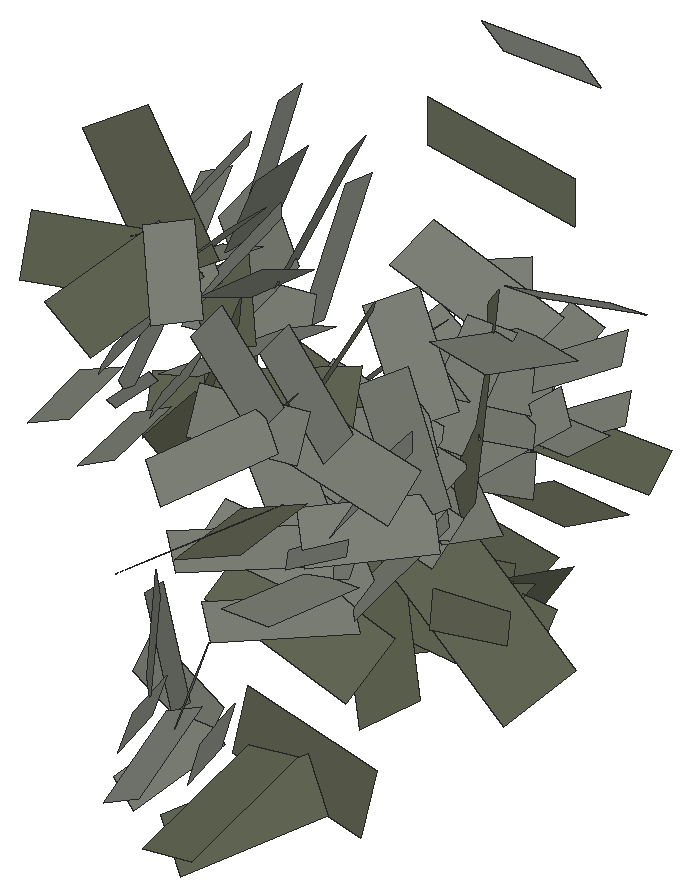
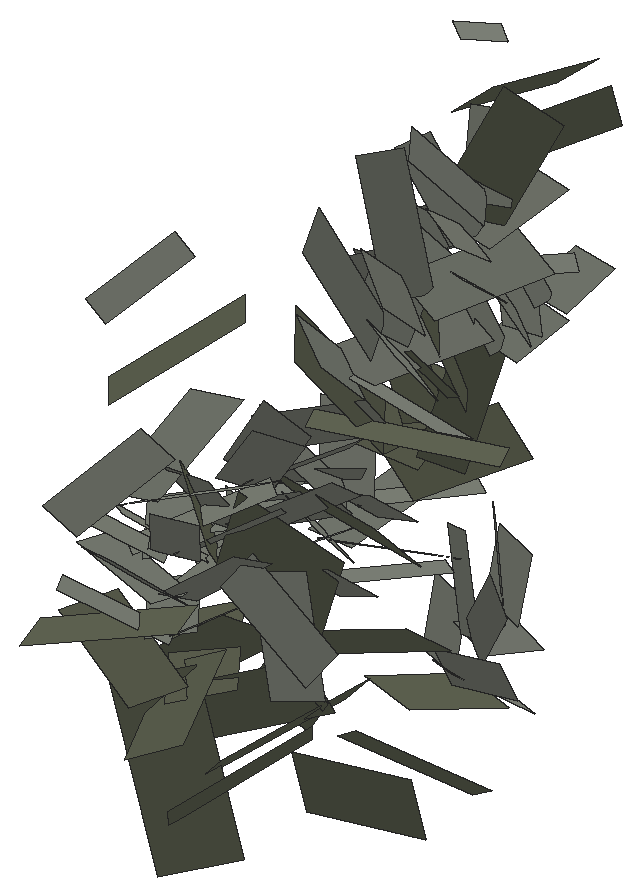
# SketchUp Ruby script. Lengths in inches.
U = 1.inch
M = Sketchup.active_model
def pt(a) = Geom::Point3d.new(a.map { |v| v * U })
def face(e, loops, mat)
  f = e.add_face(loops[0].map { |a| pt(a) })
  loops[1..].each { |l| e.add_face(l.map { |a| pt(a) }).erase! }
  f.material = f.back_material = mat if mat
  f
end
# faces: each face lists its corners as indices into pts; further lists are holes
def faces(e, pts, list, mat = nil) = list.each { |f| face(e, (f[0].is_a?(Array) ? f : [f]).map { |l| l.map { |i| pts[i] } }, mat) }
# xy, xz, yz: faces in a plane at the given z, y or x. An outline is a flat list of corners, or four numbers for a rectangle; further outlines are holes
def ring(l) = l.size == 4 ? [[l[0], l[1]], [l[2], l[1]], [l[2], l[3]], [l[0], l[3]]] : l.each_slice(2).to_a
def flat(e, list, mat, &to3) = list.each { |f| face(e, (f[0].is_a?(Array) ? f : [f]).map { |l| ring(l).map { |u, v| to3.(u, v) } }, mat) }
def xy(e, z, list, mat = nil) = flat(e, list, mat) { |x, y| [x, y, z] }
def xz(e, y, list, mat = nil) = flat(e, list, mat) { |x, z| [x, y, z] }
def yz(e, x, list, mat = nil) = flat(e, list, mat) { |y, z| [x, y, z] }
def lines(e, pts, list) = list.each { |a, b| e.add_line(pt(pts[a]), pt(pts[b])) }
# prism: a flat outline (further loops are holes) pulled along v
def prism(e, loops, v, mat = nil)
  f = face(e, loops, mat); d = Geom::Vector3d.new(v.map { |x| x * U })
  f.pushpull(f.normal.samedirection?(d) ? d.length : -d.length)
end
def box(e, o, s, mat = nil) = prism(e, [[o, [o[0] + s[0], o[1], o[2]], [o[0] + s[0], o[1] + s[1], o[2]], [o[0], o[1] + s[1], o[2]]]], [0, 0, s[2]], mat)
def at(x, y, z, deg = 0) = Geom::Transformation.translation(pt([x, y, z])) * Geom::Transformation.rotation(ORIGIN, Z_AXIS, deg.degrees)
def axes(o, x, y, z) = Geom::Transformation.new([*x, 0, *y, 0, *z, 0, *pt(o).to_a, 1])
def part(name) = M.definitions.add(name)
# library, detail: a bought-in or finely detailed component or shape, given as its bounding box
def library(name, o, s) = part(name).tap { |d| box(d.entities, o, s) }
def detail(e, o, s) = box(e.add_group.entities, o, s)
def put(e, d, t, mat = nil) = e.add_instance(d, t).tap { |i| i.material = mat if mat }
def group(e, t, mat = nil) = e.add_group.tap { |g| g.transformation = t; g.material = mat if mat }.entities
root = M.entities
M.materials.add("viburnumblaasdfas0df1w06d").color = [98, 102, 84]
M.materials.add("viburnumbladsadfasdfad0w122").color = [125, 129, 119]
c1 = part("Component\#315")
p = [[0.25,0,0],[2.05,0.01,0.35],[1.81,4.2,1.66],[0,4.19,1.3125]]
faces(c1.entities,p,[[0,1,2,3]],"viburnumbladsadfasdfad0w122")
c2 = part("viburnumblad2")
put(c2.entities,c1,axes([-19.23,-4.49,-32.18],[83.35428,0,0],[0,79.38502,0],[0,0,83.35428]))
c3 = part("Component\#314")
p = [[0.14,0,0],[2.58,0.05,0.25],[2.44,5.11,2.64],[0,5.05,2.39]]
faces(c3.entities,p,[[0,1,2,3]],"viburnumblaasdfas0df1w06d")
c4 = part("viburnumblad1\#2")
put(c4.entities,c3,axes([-37.25,6.23,19.31],[75.98784,0,0],[0,65.50676,0],[0,0,75.98784]))
put(root,c2,axes([1219.69,283.23,15.31],[0.00305,-0.01398,-0.00068],[0.01153,0.00223,0.00588],[-0.00601,-0.00193,0.01207]))
put(root,c2,axes([1222.5625,273.78,23.07],[0.00909,0.00693,0.00924],[-0.00802,0.01085,-0.00026],[-0.00757,-0.00532,0.01142]))
put(root,c2,axes([1222.37,270.28,24.57],[0.00793,0.00729,0.0045],[-0.0069,0.00732,0.00029],[-0.00293,-0.00317,0.01031]))
put(root,c2,axes([1221.25,274.45,24.79],[0.0119,-0.00385,0.00772],[-0.0001,0.01309,0.00669],[-0.00863,-0.00547,0.01057]))
put(root,c2,axes([1223.11,270.6,8.56],[0.00419,0.0043,0.00836],[-0.00938,0.00585,0.00169],[-0.00405,-0.0083,0.0063]))
put(root,c2,axes([1223.71,270.04,24.98],[-0.00696,0.00812,-0.0009],[-0.00864,-0.00777,-0.00327],[-0.00289,-0.00129,0.01072]))
put(root,c2,axes([1222.02,270.29,9.54],[0.00908,-0.00221,0.00614],[-0.004,0.00655,0.00828],[-0.00518,-0.00884,0.00448]))
put(root,c2,axes([1222.11,267.88,23.36],[-0.00916,-0.00124,-0.00492],[0.00298,-0.00959,-0.00307],[-0.00406,-0.0039,0.00779]))
put(root,c2,axes([1223.32,273.35,25.98],[-0.0119,0.00385,-0.00772],[-0.00199,-0.01402,-0.00394],[-0.0084,-0.00214,0.01187]))
put(root,c2,axes([1223.97,273.94,21.96],[0.00099,0.01426,0.00559],[-0.01157,0.00302,-0.00566],[-0.00706,-0.00428,0.01216]))
put(root,c2,axes([1221.06,268.99,22],[0.00892,-0.00552,0.00065],[0.00374,0.00694,0.00752],[-0.00413,-0.00589,0.00653]))
put(root,c4,axes([1222.82,269.56,25.68],[0.01074,0.00549,0.00552],[-0.0086,0.00502,0.01173],[0.00238,-0.01127,0.00657]))
put(root,c2,axes([1221.75,270.41,25.78],[0.0105,-0.00104,0.00371],[-0.00021,0.00971,0.00332],[-0.00385,-0.00347,0.00991]))
put(root,c4,axes([1223.4375,271.49,20.03],[0.00961,0.00314,0.00694],[-0.00599,0.01265,0.00258],[-0.0056,-0.00466,0.00986]))
put(root,c2,axes([1221.25,283.18,14.25],[-0.00599,-0.01069,-0.00483],[0.01087,-0.00815,0.00451],[-0.00654,-0.00189,0.01181]))
put(root,c2,axes([1221.54,269.65,11.03],[0.00876,-0.00688,-0.00103],[0.00337,0.00275,0.0103],[-0.00608,-0.00838,0.00422]))
put(root,c2,axes([1221.09,268.73,23.41],[0.00345,-0.00905,-0.004],[0.00865,0.00062,0.00578],[-0.00475,-0.00515,0.0067]))
put(root,c2,axes([1223.58,270.18,26.46],[-0.0105,0.00104,-0.00371],[-0.00071,-0.0111,-0.00111],[-0.00379,-0.00081,0.01049]))
put(root,c2,axes([1224.17,270.33,9.07],[-0.00914,0.00718,0.00108],[-0.00427,-0.00422,-0.00808],[-0.00509,-0.00746,0.00659]))
put(root,c2,axes([1223.05,269.15,21.66],[-0.00798,-0.00075,-0.00527],[0.00298,-0.00959,-0.00307],[-0.00502,-0.00401,0.00721]))
put(root,c2,axes([1222.11,269.23,22.6],[-0.00404,-0.00727,-0.00631],[0.00772,-0.00559,0.00142],[-0.00472,-0.00433,0.00722]))
put(root,c4,axes([1226.73,274.68,19.48],[-0.0074,0.01393,0.00333],[-0.01491,-0.00558,-0.00981],[-0.00631,-0.00654,0.01332]))
put(root,c4,axes([1224.71,267.86,26.64],[-0.0017,0.006,0.01056],[-0.01273,-0.00619,0.00147],[0.00521,-0.00927,0.00611]))
put(root,c4,axes([1223.28,272.7,17.98],[-0.00329,-0.00864,-0.00687],[0.00632,-0.00867,0.00771],[-0.00921,-0.00096,0.00528]))
put(root,c2,axes([1221.68,270.87,27.4375],[0.00725,-0.00846,0.00094],[0.00707,0.00667,0.00553],[-0.00474,-0.00299,0.00967]))
put(root,c2,axes([1223.66,269.83,10.53],[-0.00908,0.00221,-0.00614],[0.00272,-0.00885,-0.00722],[-0.00599,-0.007,0.00633]))
put(root,c2,axes([1222.98,270.5,27.85],[-0.00759,-0.00699,-0.00431],[0.00673,-0.00866,0.00218],[-0.0047,-0.00111,0.01008]))
put(root,c4,axes([1225.1875,284.26,7.73],[-0.00681,0.00895,0.00759],[-0.01184,-0.01026,0.00148],[0.00579,-0.00507,0.01117]))
put(root,c4,axes([1222.63,271.1,19.52],[0.00733,-0.00886,0.00054],[0.00689,0.00642,0.00923],[-0.00652,-0.00466,0.00706]))
put(root,c2,axes([1222.17,269.87,21.61],[0.0036,-0.00945,-0.00418],[0.00778,0.00056,0.0052],[-0.00475,-0.00515,0.0067]))
put(root,c2,axes([1222.74,269.21,11.63],[-0.00409,-0.00375,-0.00971],[0.008,-0.0078,-0.00036],[-0.00665,-0.00708,0.00553]))
put(root,c4,axes([1226.97,275.46,16.59],[0.00378,0.01126,0.01091],[-0.0152,0.00977,-0.00482],[-0.0086,-0.00789,0.01113]))
put(root,c4,axes([1226.52,275.4375,4.4375],[0.00278,0.00293,0.01264],[-0.01346,0.00734,0.00126],[-0.00579,-0.01128,0.00389]))
put(root,c2,axes([1223.2,275.33,21.99],[0.01174,-0.00298,0.00601],[-0.0001,0.01309,0.00669],[-0.00729,-0.00586,0.01134]))
put(root,c2,axes([1225.24,274.7,23.11],[-0.01142,0.0037,-0.00741],[-0.00214,-0.01514,-0.00425],[-0.0084,-0.00214,0.01187]))
put(root,c2,axes([1222.55,275.04,25.98],[-0.00095,-0.01366,-0.00535],[0.01077,-0.00429,0.00904],[-0.00996,-0.00334,0.01028]))
put(root,c4,axes([1226.56,273.37,6.2],[-0.00836,0.0066,0.00609],[-0.00962,-0.00288,-0.01008],[-0.00344,-0.01004,0.00615]))
put(root,c2,axes([1222.5,271.42,24.95],[0.0071,-0.00744,-0.0001],[0.00707,0.00667,0.00553],[-0.00393,-0.00389,0.00972]))
put(root,c2,axes([1224.97,272.57,15.58],[0.00865,0.00796,0.00491],[-0.00918,0.00854,0.00232],[-0.00184,-0.00511,0.01153]))
put(root,c2,axes([1226.24,272.74,14.17],[-0.00016,0.01206,0.00411],[-0.0133,0.00032,-0.00146],[-0.00141,-0.0041,0.01199]))
put(root,c2,axes([1222.7,270.625,10.75],[0.0033,-0.00751,-0.0076],[0.00833,-0.00317,0.00675],[-0.00669,-0.00765,0.00466]))
put(root,c4,axes([1226.85,274.35,9.74],[0.00263,0.01141,0.00764],[-0.01577,0.00377,-0.0002],[-0.00192,-0.0074,0.01171]))
put(root,c4,axes([1225.52,272.19,17.19],[-0.00905,0.00252,-0.00817],[0.0005,-0.01365,-0.00475],[-0.00803,-0.00297,0.00749]))
put(root,c2,axes([1222.67,275.69,23.86],[0.00774,-0.01238,0.00167],[0.00805,0.00648,0.01066],[-0.00962,-0.00465,0.01009]))
put(root,c4,axes([1225.64,281.85,8.35],[-0.01009,0.00576,0.00864],[-0.00958,-0.01423,-0.00203],[0.00708,-0.00619,0.01118]))
put(root,c2,axes([1222.81,271.38,26.42],[-0.00024,-0.01092,-0.00238],[0.01005,-0.00131,0.00499],[-0.0051,-0.00202,0.00975]))
put(root,c2,axes([1224.16,274.94,24.74],[-0.00909,-0.00693,-0.00924],[0.00664,-0.01276,0.00304],[-0.00946,-0.0023,0.01102]))
put(root,c2,axes([1225.72,281.88,16.11],[0.00269,0.01067,0.0031],[-0.01059,0.00139,0.00439],[0.00368,-0.00386,0.01011]))
put(root,c2,axes([1226.52,272.21,15.84],[-0.00888,0.0091,0.0009],[-0.00895,-0.0084,-0.00345],[-0.00187,-0.00303,0.01224]))
put(root,c2,axes([1226.28,282.43,14.79],[-0.00563,0.00838,0.00295],[-0.00922,-0.00664,0.00128],[0.00288,-0.0019,0.0109]))
put(root,c4,axes([1224.22,276.91,12.78],[0.00372,-0.01109,0.0102],[0.00971,0.0119,0.0094],[-0.01253,0.00356,0.00844]))
put(root,c4,axes([1225.8125,272.51,8.18],[-0.01158,0.00263,-0.00305],[0.00041,-0.00999,-0.01013],[-0.00401,-0.00833,0.00806]))
put(root,c2,axes([1223.86,271.28,10.08],[-0.00392,-0.0036,-0.00932],[0.00864,-0.00842,-0.00039],[-0.00665,-0.00708,0.00553]))
put(root,c2,axes([1226.52,277.64,16.53],[-0.00038,0.01114,0.00561],[-0.01176,-0.00241,0.0034],[0.00455,-0.00528,0.01006]))
put(root,c2,axes([1225.68,273.81,12.76],[0.00904,0.00831,0.00513],[-0.00826,0.00768,0.00209],[-0.00184,-0.00511,0.01153]))
put(root,c2,axes([1226.75,281.6,17.35],[-0.00577,0.00885,0.00437],[-0.00922,-0.00664,0.00128],[0.00353,-0.00288,0.01049]))
put(root,c2,axes([1227.46,281.66,19.6],[0,0.01516,0.00154],[-0.01516,-0.00015,0.00148],[0.00149,-0.00153,0.01509]))
put(root,c2,axes([1227.26,273.59,13.04],[-0.00853,0.00873,0.00086],[-0.00967,-0.00907,-0.00372],[-0.00187,-0.00303,0.01224]))
put(root,c4,axes([1226.25,275.82,7.68],[0.01152,0.00345,0.00714],[-0.0073,0.01349,0.00527],[-0.00481,-0.00695,0.01113]))
put(root,c4,axes([1226.02,267.25,28.4],[-0.00973,0.00003,0.00746],[-0.00524,-0.01136,-0.00678],[0.00594,-0.00739,0.00778]))
put(root,c2,axes([1227.01,278.67,15.36],[-0.00848,0.00652,0.00394],[-0.00785,-0.00971,-0.00119],[0.00311,-0.00363,0.01115]))
put(root,c2,axes([1225.46,282.06,17.8],[0.00958,0.00624,0.00001],[-0.00544,0.00834,0.00562],[0.00306,-0.00472,0.00995]))
put(root,c2,axes([1226.12,277.38,18.26],[0.00829,0.0091,0.00248],[-0.00839,0.00593,0.00669],[0.00415,-0.0063,0.00965]))
put(root,c4,axes([1224.15,272.31,18.83],[-0.001,-0.01064,-0.00433],[0.01169,-0.00333,0.00541],[-0.00539,-0.00308,0.00855]))
put(root,c4,axes([1224.46,273.3,18.27],[0.00803,-0.00983,0.00384],[0.00868,0.0101,0.00771],[-0.00745,-0.00186,0.01082]))
put(root,c2,axes([1225.12,273.74,14.22],[0.0124,-0.0008,0.00284],[-0.00048,0.01054,0.00506],[-0.0029,-0.00547,0.01114]))
put(root,c4,axes([1225.96,272.52,17.28],[-0.01126,-0.00328,-0.00424],[0.0051,-0.0131,-0.00341],[-0.00278,-0.00386,0.0103]))
put(root,c2,axes([1227.63,277.35,17.88],[-0.00883,0.00666,0.00546],[-0.00785,-0.00971,-0.00119],[0.00409,-0.00438,0.01062]))
put(root,c4,axes([1224.47,285.01,6.3],[-0.00857,-0.01458,-0.00131],[0.01562,-0.00975,0.00697],[-0.00558,0.00226,0.01502]))
put(root,c4,axes([1228.875,280.77,8.22],[0.00192,0.00886,0.01301],[-0.01818,-0.00012,0.00276],[0.00142,-0.01315,0.00875]))
put(root,c2,axes([1227.07,282.77,16.08],[-0.01085,0.00184,0.00308],[-0.00218,-0.01013,-0.00164],[0.00269,-0.00234,0.01086]))
put(root,c4,axes([1228.5625,283.3,23.73],[-0.00859,0.01076,0.00042],[-0.01222,-0.00981,0.0027],[0.00229,0.0015,0.01233]))
put(root,c2,axes([1228.73,282.02,17.72],[-0.01077,0.01075,0.00083],[-0.01084,-0.01091,0.00051],[0.00094,-0.00022,0.01521]))
put(root,c2,axes([1227.29,273.54,14.74],[-0.0124,0.0008,-0.00284],[-0.0002,-0.01247,-0.00265],[-0.00294,-0.00253,0.01214]))
put(root,c2,axes([1225.17,283.12,16.67],[0.01085,-0.00184,-0.00308],[0.00296,0.01015,0.00436],[0.00203,-0.00494,0.01011]))
put(root,c2,axes([1225.56,278.66,17.27],[0.01211,0.00173,-0.00211],[0,0.01038,0.00684],[0.00312,-0.00685,0.00964]))
put(root,c2,axes([1227.48,267.71,22.61],[0.00766,0.00322,0.00823],[-0.00853,0.00606,0.00527],[-0.00262,-0.00929,0.00521]))
put(root,c2,axes([1228.25,284.97,28.43],[-0.01136,0.00626,-0.00167],[-0.00565,-0.00941,0.00229],[-0.00013,0.00352,0.01104]))
put(root,c4,axes([1226.22,284.82,10.25],[-0.01133,-0.00353,0.00405],[0.00312,-0.01382,-0.0033],[0.00465,-0.0017,0.01152]))
put(root,c2,axes([1228.58,273.32,17.38],[0.00252,0.00942,0.00914],[-0.01307,0.00092,0.00265],[0.00124,-0.00944,0.00938]))
put(root,c2,axes([1228.74,268.35,21.75],[-0.00034,0.00733,0.00907],[-0.01154,0.00172,-0.00184],[-0.00225,-0.00876,0.00608]))
put(root,c2,axes([1228.71,275.44,14.99],[0.00219,0.00955,0.00743],[-0.01307,0.00092,0.00265],[0.0015,-0.00837,0.01031]))
put(root,c4,axes([1227.9375,277.94,14.21],[0.01183,-0.00442,0.01203],[-0.00182,0.01827,0.0085],[-0.01272,-0.00605,0.01028]))
put(root,c2,axes([1228.88,267.21,22.73],[-0.00814,0.00715,0.0046],[-0.00805,-0.00423,-0.00746],[-0.00268,-0.00803,0.00677]))
put(root,c2,axes([1226.69,283.58,15],[-0.01,-0.00652,-0.00001],[0.00542,-0.00831,-0.00274],[0.00166,-0.00256,0.01102]))
put(root,c2,axes([1225.22,274.05,16.15],[0.00888,-0.0091,-0.0009],[0.00823,0.00741,0.00631],[-0.00398,-0.00497,0.01104]))
put(root,c2,axes([1227.6875,278.94,16.84],[-0.01211,-0.00173,0.00211],[0.00069,-0.01077,-0.00395],[0.00303,-0.00413,0.011]))
put(root,c2,axes([1226.67,266.04,31.06],[-0.00866,-0.00577,-0.00263],[0.00674,-0.00675,-0.0074],[0.00215,-0.00706,0.0084]))
put(root,c2,axes([1227.87,274.84,16.45],[0.01106,0.0052,0.00541],[-0.00756,0.007,0.00872],[0.00055,-0.01018,0.00865]))
put(root,c2,axes([1226.76,273.69,16.42],[-0.00865,-0.00796,-0.00491],[0.00846,-0.00952,0.00054],[-0.00401,-0.0029,0.01175]))
put(root,c2,axes([1225.34,283.9375,15.39],[0.00554,-0.00849,-0.00419],[0.01058,0.00621,0.0014],[0.00119,-0.0044,0.01049]))
put(root,c2,axes([1225.8,275.05,13.33],[0.00852,-0.00783,-0.00192],[0.00823,0.00741,0.00631],[-0.003,-0.00593,0.01088]))
put(root,c4,axes([1230.76,284.66,14.06],[-0.00473,0.01294,-0.00003],[-0.01473,-0.00539,-0.00308],[-0.0025,-0.00088,0.01352]))
put(root,c2,axes([1229.72,274.57,16.21],[-0.00749,0.00812,0.00752],[-0.01012,-0.00577,-0.00385],[0.00099,-0.00855,0.01022]))
put(root,c2,axes([1228.74,269.74,21.22],[0.00736,0.00309,0.0079],[-0.00921,0.00654,0.0057],[-0.00262,-0.00929,0.00521]))
put(root,c4,axes([1226.46,282.15,11.18],[-0.0111,-0.00766,0.00199],[0.00742,-0.01279,-0.00569],[0.00489,-0.00308,0.01206]))
put(root,c2,axes([1225.56,279.84,16.14],[0.00848,-0.00639,-0.00524],[0.0093,0.00903,0.00402],[0.00207,-0.0066,0.01002]))
put(root,c2,axes([1227.32,282.89,17.67],[-0.00958,-0.00624,-0.00001],[0.00602,-0.00923,-0.00305],[0.00166,-0.00256,0.01102]))
put(root,c2,axes([1229.35,285.76,20.19],[-0.01136,0.00239,-0.0048],[-0.00314,-0.01208,0.00143],[-0.00434,0.00249,0.01152]))
put(root,c2,axes([1227.1,279.92,15.85],[-0.00866,-0.0095,-0.00259],[0.00823,-0.00655,-0.00374],[0.002,-0.00468,0.01099]))
put(root,c2,axes([1229.03,282.76,19.75],[-0.01523,0.00004,-0.00037],[-0.00005,-0.01523,0.00032],[-0.00037,0.00032,0.01523]))
put(root,c4,axes([1225.83,284.96,12.55],[-0.00529,-0.01137,-0.00003],[0.01295,-0.00601,-0.0028],[0.00218,-0.00104,0.01231]))
put(root,c2,axes([1226.03,283.35,18.125],[0.00577,-0.00885,-0.00437],[0.0098,0.00575,0.0013],[0.00119,-0.0044,0.01049]))
put(root,c2,axes([1226.3,283.75,16.6],[-0.00269,-0.01067,-0.0031],[0.01162,-0.00239,-0.00186],[0.00104,-0.00341,0.01086]))
put(root,c4,axes([1230.4,278.04,8.43],[0.00636,0.01278,0.00656],[-0.01653,0.00548,0.00535],[0.00178,-0.00782,0.01351]))
